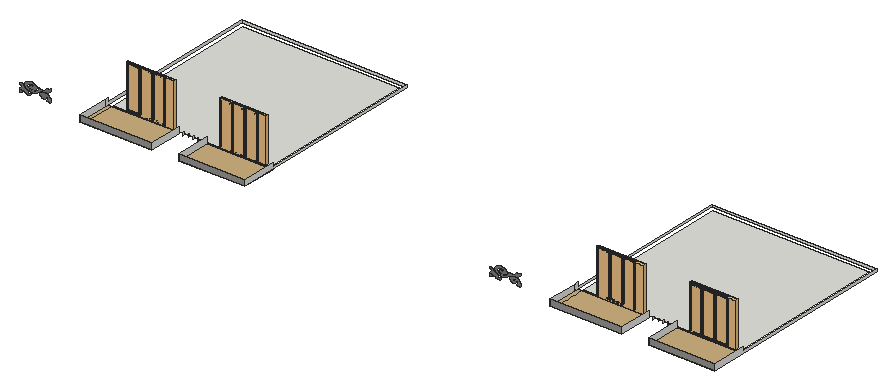
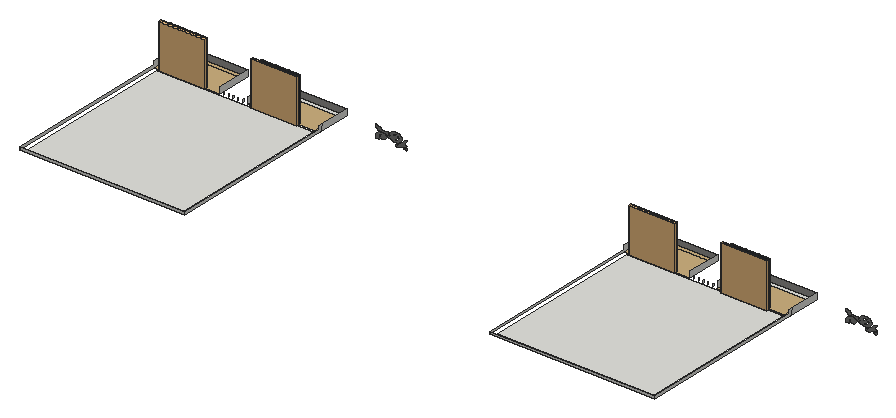
# SketchUp Ruby script. Lengths in inches.
U = 1.inch
M = Sketchup.active_model
def pt(a) = Geom::Point3d.new(a.map { |v| v * U })
def face(e, loops, mat)
  f = e.add_face(loops[0].map { |a| pt(a) })
  loops[1..].each { |l| e.add_face(l.map { |a| pt(a) }).erase! }
  f.material = f.back_material = mat if mat
  f
end
# faces: each face lists its corners as indices into pts; further lists are holes
def faces(e, pts, list, mat = nil) = list.each { |f| face(e, (f[0].is_a?(Array) ? f : [f]).map { |l| l.map { |i| pts[i] } }, mat) }
# xy, xz, yz: faces in a plane at the given z, y or x. An outline is a flat list of corners, or four numbers for a rectangle; further outlines are holes
def ring(l) = l.size == 4 ? [[l[0], l[1]], [l[2], l[1]], [l[2], l[3]], [l[0], l[3]]] : l.each_slice(2).to_a
def flat(e, list, mat, &to3) = list.each { |f| face(e, (f[0].is_a?(Array) ? f : [f]).map { |l| ring(l).map { |u, v| to3.(u, v) } }, mat) }
def xy(e, z, list, mat = nil) = flat(e, list, mat) { |x, y| [x, y, z] }
def xz(e, y, list, mat = nil) = flat(e, list, mat) { |x, z| [x, y, z] }
def yz(e, x, list, mat = nil) = flat(e, list, mat) { |y, z| [x, y, z] }
def lines(e, pts, list) = list.each { |a, b| e.add_line(pt(pts[a]), pt(pts[b])) }
# prism: a flat outline (further loops are holes) pulled along v
def prism(e, loops, v, mat = nil)
  f = face(e, loops, mat); d = Geom::Vector3d.new(v.map { |x| x * U })
  f.pushpull(f.normal.samedirection?(d) ? d.length : -d.length)
end
def box(e, o, s, mat = nil) = prism(e, [[o, [o[0] + s[0], o[1], o[2]], [o[0] + s[0], o[1] + s[1], o[2]], [o[0], o[1] + s[1], o[2]]]], [0, 0, s[2]], mat)
def at(x, y, z, deg = 0) = Geom::Transformation.translation(pt([x, y, z])) * Geom::Transformation.rotation(ORIGIN, Z_AXIS, deg.degrees)
def axes(o, x, y, z) = Geom::Transformation.new([*x, 0, *y, 0, *z, 0, *pt(o).to_a, 1])
def part(name) = M.definitions.add(name)
# library, detail: a bought-in or finely detailed component or shape, given as its bounding box
def library(name, o, s) = part(name).tap { |d| box(d.entities, o, s) }
def detail(e, o, s) = box(e.add_group.entities, o, s)
def put(e, d, t, mat = nil) = e.add_instance(d, t).tap { |i| i.material = mat if mat }
def group(e, t, mat = nil) = e.add_group.tap { |g| g.transformation = t; g.material = mat if mat }.entities
root = M.entities
M.materials.add("Wine2").color = [0, 0, 0]
M.materials["Wine2"].alpha = 0
M.materials.add("[0043_SaddleBrown]4").color = [124, 123, 122]
M.materials.add("[0130_Gainsboro]").color = [39, 45, 50]
M.materials.add("[Granite Light Gray]").color = [149, 148, 144]
M.materials.add("[Wood Floor Light]").color = [204, 176, 127]
c1 = part("Framed glazing panel")
xy(c1.entities,0,[[0,-0.98,43.07,0],[0,0,43.07,1.4]],"[0130_Gainsboro]")
xy(c1.entities,0.3,[[0.3,-1.43,42.77,-0.98]],"[0130_Gainsboro]")
xy(c1.entities,2.95,[[2.95,-1.43,40.12,-0.63],[2.95,-0.63,40.12,0],[2.95,0,40.12,0.64],[2.95,0.64,40.12,1.4]],"[0130_Gainsboro]")
xy(c1.entities,3.54,[[3.54,-0.63,39.53,0],[3.54,0,39.53,0.64]],"[0130_Gainsboro]")
xy(c1.entities,111.8125,[[3.54,-0.63,39.53,0],[3.54,0,39.53,0.64]],"[0130_Gainsboro]")
xy(c1.entities,112.4,[[2.95,-1.43,40.12,-0.63],[2.95,-0.63,40.12,0],[2.95,0,40.12,0.64],[2.95,0.64,40.12,1.4]],"[0130_Gainsboro]")
xy(c1.entities,115.05,[[0.3,-1.43,42.77,-0.98]],"[0130_Gainsboro]")
xy(c1.entities,115.35,[[0,-0.98,43.07,0],[0,0,43.07,1.4]],"[0130_Gainsboro]")
xz(c1.entities,-1.43,[[[0.3,0.3,42.77,115.05],[2.95,2.95,40.12,112.4]]],"[0130_Gainsboro]")
xz(c1.entities,-0.98,[[[0,0,43.07,115.35],[0.3,0.3,42.77,115.05]]],"[0130_Gainsboro]")
xz(c1.entities,-0.63,[[[2.95,2.95,40.12,112.4],[3.54,3.54,39.53,111.8125]]],"[0130_Gainsboro]")
xz(c1.entities,0,[[3.54,3.54,39.53,111.8125]],"Wine2")
xz(c1.entities,0,[[[0,0,43.07,115.35],[2.95,2.95,40.12,112.4]],[[2.95,2.95,40.12,112.4],[3.54,3.54,39.53,111.8125]]],"[0130_Gainsboro]")
xz(c1.entities,0.64,[[[2.95,2.95,40.12,112.4],[3.54,3.54,39.53,111.8125]]],"[0130_Gainsboro]")
xz(c1.entities,1.4,[[[0,0,43.07,115.35],[2.95,2.95,40.12,112.4]]],"[0130_Gainsboro]")
yz(c1.entities,0,[[-0.98,0,0,115.35],[0,0,1.4,115.35]],"[0130_Gainsboro]")
yz(c1.entities,0.3,[[-1.43,0.3,-0.98,115.05]],"[0130_Gainsboro]")
yz(c1.entities,2.95,[[-1.43,2.95,-0.63,112.4],[-0.63,2.95,0,112.4],[0,2.95,0.64,112.4],[0.64,2.95,1.4,112.4]],"[0130_Gainsboro]")
yz(c1.entities,3.54,[[-0.63,3.54,0,111.8125],[0,3.54,0.64,111.8125]],"[0130_Gainsboro]")
yz(c1.entities,39.53,[[-0.63,3.54,0,111.8125],[0,3.54,0.64,111.8125]],"[0130_Gainsboro]")
yz(c1.entities,40.12,[[-1.43,2.95,-0.63,112.4],[-0.63,2.95,0,112.4],[0,2.95,0.64,112.4],[0.64,2.95,1.4,112.4]],"[0130_Gainsboro]")
yz(c1.entities,42.77,[[-1.43,0.3,-0.98,115.05]],"[0130_Gainsboro]")
yz(c1.entities,43.07,[[-0.98,0,0,115.35],[0,0,1.4,115.35]],"[0130_Gainsboro]")
c2 = part("Glazing assembly")
put(c2.entities,c1,axes([90.57,1.43,0],[1.05148,0,0],[0,1,0],[0,0,1]))
put(c2.entities,c1,axes([0,1.43,0],[1.05148,0,0],[0,1,0],[0,0,1]))
put(c2.entities,c1,axes([45.29,1.43,0],[1.05148,0,0],[0,1,0],[0,0,1]))
c3 = library("Curtains",[0,0,0],[121.73,8.19,117.22])
xy(root,640.875,[[602.01,651.03,703.26,657.03],[849.76,651.03,951.01,657.03],[1852.64,651.03,1953.89,657.03],[2100.38,651.03,2201.63,657.03]])
xy(root,646.4375,[[551.76,559.875,742.44,570.83],[1802.38,559.875,1993.07,570.83],[563.08,657.03,978.86,1085.17],[1813.71,657.03,2229.49,1085.17]])
xy(root,646.4375,[[814.89,559.875,990.19,570.83],[2065.52,559.875,2240.81,570.83],[551.76,570.83,563.08,651.03],[563.08,570.83,742.44,651.03],[814.89,570.83,978.86,651.03],
  [978.86,570.83,990.19,651.03],[1802.38,570.83,1813.71,651.03],[1813.71,570.83,1993.07,651.03],[2065.52,570.83,2229.49,651.03],[2229.49,570.83,2240.81,651.03]],"[Wood Floor Light]")
xz(root,559.875,[[551.76,646.4375,742.44,662.4375],[814.89,646.4375,990.19,662.4375],[1802.38,646.4375,1993.07,662.4375],[2065.52,646.4375,2240.81,662.4375]],"[Granite Light Gray]")
xz(root,589.17,[[368.68,640.49,369.04,640.8,369.43,641.09,369.84,641.36,370.29,641.62,370.77,641.85,371.27,642.07,371.79,642.26,372.34,642.43,372.9,642.58,373.48,642.71,374.07,642.81,374.67,642.89,374.3,643.17,373.9,643.4375,373.47,643.68,373.02,643.91,372.54,644.125,372.03,644.3125,371.51,644.48,370.97,644.62,370.41,644.74,369.85,644.83,369.27,644.9,368.68,644.94],[1619.31,640.49,1619.66,640.8,1620.05,641.09,1620.47,641.36,1620.92,641.62,1621.39,641.85,1621.9,642.07,1622.42,642.26,1622.96,642.43,1623.52,642.58,1624.1,642.71,1624.69,642.81,1625.29,642.89,1624.92,643.17,1624.53,643.4375,1624.1,643.68,1623.64,643.91,1623.16,644.125,1622.66,644.3125,1622.14,644.48,1621.6,644.62,1621.04,644.74,1620.47,644.83,1619.89,644.9,1619.31,644.94],[392.33,641.03,393.35,641.04,394.16,641.12,394.92,641.3125,395.6,641.61,396.15,641.99,396.54,642.43,396.76,642.92,396.8,643.43,396.65,643.93,396.32,644.39,395.83,644.8,395.21,645.13,394.48,645.37,394.37,644.86,394.05,644.38,393.54,643.98,392.875,643.66,392.1,643.47,391.27,643.4,390.45,643.47,389.67,643.66,389.01,643.98,388.5,644.38,388.18,644.86,388.07,645.37,388.03,645.77,388,646.18,387.99,646.58,388,646.99,388.03,647.39,388.07,647.8,388.14,648.2,388.22,648.6,388.3125,649,388.43,649.4,388.5625,649.8,388.71,650.19,387.25,650.55,385.84,650.99,384.48,651.48,383.2,652.05,381.99,652.67,380.87,653.35,379.84,654.09,378.91,654.87,378.08,655.69,377.37,656.56,376.76,657.45,376.27,658.375,375.75,658.8,375.2,659.22,374.64,659.625,374.05,660.02,373.44,660.41,372.81,660.78,372.17,661.14,371.51,661.49,370.82,661.82,370.125,662.14,369.41,662.45,368.68,662.74,368.68,660.01,369.7,659.23,370.56,658.39,371.24,657.48,371.73,656.53,372.03,655.56,372.13,654.5625,372.03,653.57,371.73,652.59,371.24,651.64,370.56,650.74,369.7,649.89,368.68,649.12,368.68,648.22,369.97,648.05,371.24,647.85,372.49,647.6,373.72,647.32,374.93,647,376.1,646.63,377.24,646.23,378.35,645.8,379.42,645.33,380.44,644.82,381.42,644.28,382.36,643.71,383.09,643.28,383.86,642.88,384.69,642.51,385.55,642.18,386.45,641.89,387.375,641.64,388.33,641.43,389.3125,641.26,390.31,641.14,391.32,641.0625],[1642.95,641.03,1643.97,641.04,1644.79,641.12,1645.55,641.3125,1646.22,641.61,1646.77,641.99,1647.17,642.43,1647.39,642.92,1647.43,643.43,1647.28,643.93,1646.95,644.39,1646.46,644.8,1645.83,645.13,1645.1,645.37,1644.99,644.86,1644.67,644.38,1644.16,643.98,1643.5,643.66,1642.73,643.47,1641.9,643.4,1641.07,643.47,1640.3,643.66,1639.63,643.98,1639.125,644.38,1638.81,644.86,1638.7,645.37,1638.65,645.77,1638.625,646.18,1638.62,646.58,1638.63,646.99,1638.65,647.39,1638.7,647.8,1638.76,648.2,1638.84,648.6,1638.9375,649,1639.05,649.4,1639.1875,649.8,1639.34,650.19,1637.875,650.55,1636.46,650.99,1635.11,651.48,1633.83,652.05,1632.62,652.67,1631.5,653.35,1630.47,654.09,1629.54,654.87,1628.71,655.69,1627.99,656.56,1627.39,657.45,1626.9,658.375,1626.375,658.8,1625.83,659.22,1625.26,659.625,1624.67,660.02,1624.07,660.41,1623.44,660.78,1622.79,661.14,1622.13,661.49,1621.45,661.82,1620.75,662.14,1620.04,662.45,1619.31,662.74,1619.31,660.01,1620.33,659.23,1621.18,658.39,1621.86,657.48,1622.36,656.53,1622.66,655.56,1622.76,654.5625,1622.66,653.57,1622.36,652.59,1621.86,651.64,1621.18,650.74,1620.33,649.89,1619.31,649.12,1619.31,648.22,1620.59,648.05,1621.87,647.85,1623.12,647.6,1624.35,647.32,1625.55,647,1626.73,646.63,1627.87,646.23,1628.97,645.8,1630.04,645.33,1631.07,644.82,1632.05,644.28,1632.98,643.71,1633.71,643.28,1634.49,642.88,1635.31,642.51,1636.17,642.18,1637.07,641.89,1638,641.64,1638.96,641.43,1639.9375,641.26,1640.93,641.14,1641.94,641.0625],[449.07,642.71,449.07,650.32,448.71,650.87,448.33,651.42,447.93,651.96,447.52,652.5,447.1,653.03,446.65,653.5625,446.2,654.09,445.72,654.61,445.24,655.12,444.74,655.63,444.22,656.13,443.69,656.63,442.83,657.33,441.85,657.96,440.75,658.52,439.5625,659,438.29,659.39,436.95,659.6875,435.56,659.89,434.14,659.99,432.72,659.99,431.31,659.89,429.92,659.69,428.58,659.39,426.64,658.73,424.95,657.86,423.5625,656.81,422.53,655.61,421.9,654.31,421.68,652.96,421.9,651.61,422.53,650.31,423.5625,649.11,424.95,648.05,426.64,647.18,428.58,646.53,429.22,646.3,429.91,646.13,430.64,646.04,431.38,646.01,432.12,646.0625,432.84,646.18,433.52,646.37,434.14,646.62,434.68,646.93,435.15,647.28,435.51,647.68,435.77,648.11,436.13,648.49,436.41,648.9,436.58,649.33,436.66,649.77,436.63,650.21,436.51,650.64,436.29,651.0625,435.97,651.46,435.5625,651.82,435.08,652.15,434.52,652.43,433.91,652.66,433.55,652.54,433.21,652.41,432.88,652.27,432.57,652.11,432.28,651.94,432.01,651.76,431.76,651.57,431.54,651.37,431.33,651.15,431.15,650.93,431,650.71,430.87,650.47,430.1,650.76,429.4375,651.12,428.89,651.56,428.49,652.05,428.24,652.57,428.16,653.12,428.24,653.67,428.49,654.19,428.89,654.68,429.4375,655.12,430.1,655.48,430.87,655.77,431.8,655.79,432.73,655.77,433.66,655.7,434.58,655.6,435.48,655.45,436.36,655.26,437.22,655.03,438.04,654.76,438.84,654.46,439.59,654.12,440.3,653.75,440.96,653.34,441.54,652.56,442.01,651.75,442.36,650.91,442.58,650.07,442.68,649.21,442.65,648.35,442.5,647.49,442.22,646.65,441.82,645.82,441.3,645.03,440.67,644.26,439.92,643.53,440.68,643.69,441.47,643.8125,442.26,643.89,443.07,643.93,443.87,643.92,444.67,643.87,445.47,643.78,446.24,643.64,447,643.47,447.72,643.25,448.42,643],
  [1699.7,642.71,1699.7,650.32,1699.33,650.87,1698.95,651.42,1698.56,651.96,1698.15,652.5,1697.72,653.03,1697.28,653.5625,1696.82,654.09,1696.35,654.61,1695.86,655.12,1695.36,655.63,1694.85,656.13,1694.32,656.63,1693.46,657.33,1692.48,657.96,1691.38,658.52,1690.1875,659,1688.91,659.39,1687.57,659.6875,1686.18,659.89,1684.77,659.99,1683.35,659.99,1681.93,659.89,1680.54,659.69,1679.2,659.39,1677.27,658.73,1675.58,657.86,1674.1875,656.81,1673.16,655.61,1672.52,654.31,1672.31,652.96,1672.52,651.61,1673.16,650.31,1674.1875,649.11,1675.58,648.05,1677.27,647.18,1679.2,646.53,1679.85,646.3,1680.54,646.13,1681.26,646.04,1682.01,646.01,1682.75,646.0625,1683.46,646.18,1684.14,646.37,1684.76,646.62,1685.31,646.93,1685.77,647.28,1686.14,647.68,1686.39,648.11,1686.76,648.49,1687.03,648.9,1687.21,649.33,1687.28,649.77,1687.26,650.21,1687.13,650.64,1686.91,651.0625,1686.59,651.46,1686.1875,651.82,1685.7,652.15,1685.15,652.43,1684.53,652.66,1684.18,652.54,1683.84,652.41,1683.51,652.27,1683.2,652.11,1682.91,651.94,1682.64,651.76,1682.39,651.57,1682.16,651.37,1681.96,651.15,1681.78,650.93,1681.62,650.71,1681.49,650.47,1680.73,650.76,1680.0625,651.12,1679.52,651.56,1679.11,652.05,1678.87,652.57,1678.78,653.12,1678.87,653.67,1679.11,654.19,1679.52,654.68,1680.0625,655.12,1680.73,655.48,1681.49,655.77,1682.43,655.79,1683.36,655.77,1684.29,655.7,1685.2,655.6,1686.11,655.45,1686.99,655.26,1687.84,655.03,1688.67,654.76,1689.46,654.46,1690.21,654.12,1690.92,653.75,1691.58,653.34,1692.17,652.56,1692.64,651.75,1692.98,650.91,1693.21,650.07,1693.31,649.21,1693.28,648.35,1693.125,647.49,1692.85,646.65,1692.44,645.82,1691.92,645.03,1691.29,644.26,1690.55,643.53,1691.31,643.69,1692.09,643.8125,1692.89,643.89,1693.69,643.93,1694.5,643.92,1695.3,643.87,1696.09,643.78,1696.87,643.64,1697.62,643.47,1698.35,643.25,1699.04,643],[399.36,650.01,402.52,650.11,405.6,650.55,408.52,651.29,411.19,652.33,413.54,653.63,415.5,655.16,416.04,655.79,416.63,656.41,417.27,657.01,417.95,657.59,418.67,658.15,419.44,658.6875,420.25,659.2,421.1,659.69,421.98,660.16,422.9,660.6,423.85,661.01,424.83,661.4,426.13,661.78,427.47,662.11,428.83,662.4,430.22,662.65,431.625,662.84,433.05,662.99,434.48,663.09,435.92,663.14,437.36,663.14,438.8,663.1,440.23,663,441.66,662.86,442.21,663.4,442.78,663.94,443.36,664.48,443.95,665.01,444.55,665.54,445.17,666.0625,445.79,666.58,447.07,667.6,447.73,668.1,448.4,668.59,449.07,669.09,449.07,674.83,448.71,674.24,448.21,673.68,447.59,673.17,446.86,672.72,446.04,672.34,445.13,672.04,444.17,671.81,443.16,671.67,442.13,671.62,441.1,671.65,440.09,671.78,439.12,671.99,438.67,670.62,437.86,669.32,436.69,668.13,435.22,667.08,433.47,666.19,431.5,665.51,429.37,665.04,427.13,664.8,424.87,664.79,422.64,665.03,420.5,665.49,418.53,666.17,418.47,664.45,418,662.75,417.14,661.12,415.89,659.57,414.3,658.15,412.39,656.89,410.2,655.82,407.79,654.95,405.1875,654.3,402.46,653.89,399.67,653.73,396.87,653.82,394.42,654.4375,392.2,655.33,390.31,656.48,388.82,657.82,387.77,659.32,387.22,660.91,387.18,662.54,387.64,664.14,388.61,665.66,390.03,667.03,391.86,668.21,394.02,669.15,395.41,669.53,396.91,669.73,398.43,669.73,399.93,669.55,401.33,669.18,402.58,668.64,403.625,667.96,404.42,667.16,404.9375,666.28,405.15,665.35,405.05,664.42,404.65,663.52,404.37,663.1875,403.99,662.89,403.53,662.65,403,662.48,402.42,662.37,401.81,662.33,401.21,662.37,400.63,662.48,400.1,662.65,399.64,662.89,399.26,663.1875,398.98,663.52,398.84,663.71,398.68,663.89,398.5,664.07,398.29,664.24,398.06,664.39,397.81,664.53,397.54,664.66,397.25,664.78,396.95,664.88,396.64,664.97,396.32,665.04,395.99,665.09,395.41,664.88,394.875,664.63,394.39,664.34,393.97,664.01,393.62,663.66,393.34,663.28,393.14,662.89,393.02,662.48,392.98,662.07,393.02,661.65,393.15,661.25,393.36,660.85,393.75,660.32,394.23,659.82,394.79,659.36,395.43,658.93,396.15,658.55,396.92,658.21,397.75,657.94,398.63,657.71,399.54,657.55,400.47,657.44,401.41,657.4,402.36,657.42,403.85,657.57,405.3,657.83,406.67,658.22,407.95,658.71,409.12,659.3,410.14,659.98,411.01,660.74,411.7,661.56,412.21,662.4375,412.53,663.35,412.65,664.27,412.56,665.2,411.95,666.59,411.03,667.91,409.8125,669.15,408.32,670.26,406.59,671.23,404.64,672.04,402.54,672.67,400.3,673.12,397.99,673.36,395.64,673.4,393.3125,673.23,391.04,672.86,388.85,671.94,386.87,670.85,385.13,669.61,383.67,668.25,382.51,666.77,381.67,665.22,381.17,663.62,381.01,661.99,381.1875,660.36,381.71,658.76,382.57,657.21,383.74,655.74,385.55,654.15,387.77,652.76,390.34,651.63,393.18,650.78,396.21,650.23],[1649.98,650.01,1653.14,650.11,1656.22,650.55,1659.14,651.29,1661.82,652.33,1664.17,653.63,1666.125,655.16,1666.67,655.79,1667.26,656.41,1667.89,657.01,1668.57,657.59,1669.3,658.15,1670.07,658.6875,1670.875,659.2,1671.72,659.69,1672.6,660.16,1673.52,660.6,1674.47,661.01,1675.46,661.4,1676.76,661.78,1678.09,662.11,1679.46,662.4,1680.84,662.65,1682.25,662.84,1683.67,662.99,1685.1,663.09,1686.54,663.14,1687.99,663.14,1689.43,663.1,1690.86,663,1692.28,662.86,1692.84,663.4,1693.41,663.94,1693.99,664.48,1694.58,665.01,1695.18,665.54,1695.79,666.0625,1696.42,666.58,1697.05,667.09,1697.7,667.6,1698.35,668.1,1699.02,668.59,1699.7,669.09,1699.7,674.83,1699.33,674.24,1698.83,673.68,1698.21,673.17,1697.49,672.72,1696.66,672.34,1695.76,672.04,1694.79,671.81,1693.79,671.67,1692.76,671.62,1691.73,671.65,1690.72,671.78,1689.74,671.99,1689.3,670.62,1688.48,669.32,1687.32,668.13,1685.84,667.08,1684.09,666.19,1682.12,665.51,1679.99,665.04,1677.76,664.8,1675.49,664.79,1673.26,665.03,1671.13,665.49,1669.15,666.17,1669.09,664.45,1668.625,662.75,1667.76,661.12,1666.52,659.57,1664.93,658.15,1663.02,656.89,1660.83,655.82,1658.41,654.95,1655.8125,654.3,1653.09,653.89,1650.3,653.73,1647.5,653.82,1645.04,654.4375,1642.83,655.33,1640.94,656.48,1639.44,657.82,1638.4,659.32,1637.84,660.91,1637.8,662.54,1638.27,664.14,1639.23,665.66,1640.65,667.03,1642.48,668.21,1644.64,669.15,1646.04,669.53,1647.53,669.73,1649.06,669.73,1650.55,669.55,1651.95,669.18,1653.2,668.64,1654.25,667.96,1655.05,667.16,1655.5625,666.28,1655.78,665.35,1655.68,664.42,1655.27,663.52,1655,663.1875,1654.62,662.89,1654.15,662.65,1653.62,662.48,1653.04,662.37,1652.44,662.33,1651.84,662.37,1651.26,662.48,1650.72,662.65,1650.26,662.89,1649.88,663.1875,1649.61,663.52,1649.47,663.71,1649.31,663.89,1649.12,664.07,1648.91,664.24,1648.68,664.39,1648.43,664.53,1648.16,664.66,1647.88,664.78,1647.58,664.88,1647.27,664.97,1646.94,665.04,1646.61,665.09,1646.03,664.88,1645.5,664.63,1645.02,664.34,1644.6,664.01,1644.25,663.66,1643.97,663.28,1643.77,662.89,1643.65,662.48,1643.61,662.07,1643.65,661.65,1643.78,661.25,1643.98,660.85,1644.37,660.32,1644.85,659.82,1645.42,659.36,1646.06,658.93,1646.77,658.55,1647.55,658.21,1648.38,657.94,1649.25,657.71,1650.16,657.55,1651.09,657.44,1652.04,657.4,1652.98,657.42,1654.47,657.57,1655.92,657.83,1657.3,658.22,1658.58,658.71,1659.74,659.3,1660.77,659.98,1661.63,660.74,1662.33,661.56,1662.84,662.4375,1663.15,663.35,1663.27,664.27,1663.18,665.2,1662.58,666.59,1661.66,667.91,1660.4375,669.15,1658.94,670.26,1657.21,671.23,1655.27,672.04,1653.16,672.67,1650.93,673.12,1648.61,673.36,1646.27,673.4,1643.9375,673.23,1641.67,672.86,1639.47,671.94,1637.49,670.85,1635.76,669.61,1634.3,668.25,1633.14,666.77,1632.3,665.22,1631.79,663.62,1631.63,661.99,1631.8125,660.36,1632.34,658.76,1633.19,657.21,1634.37,655.74,1636.17,654.15,1638.39,652.76,1640.96,651.63,1643.8,650.78,1646.84,650.23]],"[0043_SaddleBrown]4")
xz(root,1096.5,[[551.76,646.4375,990.19,652.4375],[1802.38,646.4375,2240.81,652.4375]])
yz(root,551.76,[[559.875,646.4375,640.11,662.4375],[640.11,646.4375,640.11,662.4375,651.03,662.4375,651.03,652.4375,1096.5,652.4375,1096.5,646.4375]])
yz(root,742.44,[[559.875,646.4375,647.91,662.4375]])
yz(root,755.44,[[647.91,646.4375,651.03,652.4375]])
yz(root,768.19,[[648.85,646.4375,651.03,652.4375]])
yz(root,780.32,[[648.85,646.4375,651.03,652.4375]])
yz(root,792.69,[[648.85,646.4375,651.03,652.4375]])
yz(root,805.57,[[648.85,646.4375,651.03,652.4375]])
yz(root,814.89,[[559.875,646.4375,651.03,662.4375]])
yz(root,990.19,[[559.875,646.4375,1096.5,646.4375,1096.5,652.4375,651.03,652.4375,651.03,662.4375,559.875,662.4375]])
yz(root,1802.38,[[559.875,646.4375,640.11,662.4375],[640.11,646.4375,640.11,662.4375,651.03,662.4375,651.03,652.4375,1096.5,652.4375,1096.5,646.4375]])
yz(root,1993.07,[[559.875,646.4375,647.91,662.4375]])
yz(root,2006.07,[[647.91,646.4375,651.03,652.4375]])
yz(root,2018.82,[[648.85,646.4375,651.03,652.4375]])
yz(root,2030.94,[[648.85,646.4375,651.03,652.4375]])
yz(root,2043.32,[[648.85,646.4375,651.03,652.4375]])
yz(root,2056.19,[[648.85,646.4375,651.03,652.4375]])
yz(root,2065.52,[[559.875,646.4375,651.03,662.4375]])
yz(root,2240.81,[[559.875,646.4375,1096.5,646.4375,1096.5,652.4375,651.03,652.4375,651.03,662.4375,559.875,662.4375]])
put(root,c2,axes([602.01,651.74,649.48],[0.75,0,0],[0,0.75,0],[0,0,1.01765]))
put(root,c3,at(604.34,651.74,646.65))
put(root,c2,axes([849.11,651.03,649.48],[0.75,0,0],[0,0.75,0],[0,0,1.01765]))
put(root,c3,at(849.76,651.03,649.66))
put(root,c2,axes([1852.64,651.74,649.48],[0.75,0,0],[0,0.75,0],[0,0,1.01765]))
put(root,c3,at(1854.97,651.74,646.65))
put(root,c2,axes([2099.73,651.03,649.48],[0.75,0,0],[0,0.75,0],[0,0,1.01765]))
put(root,c3,at(2100.38,651.03,649.66))
